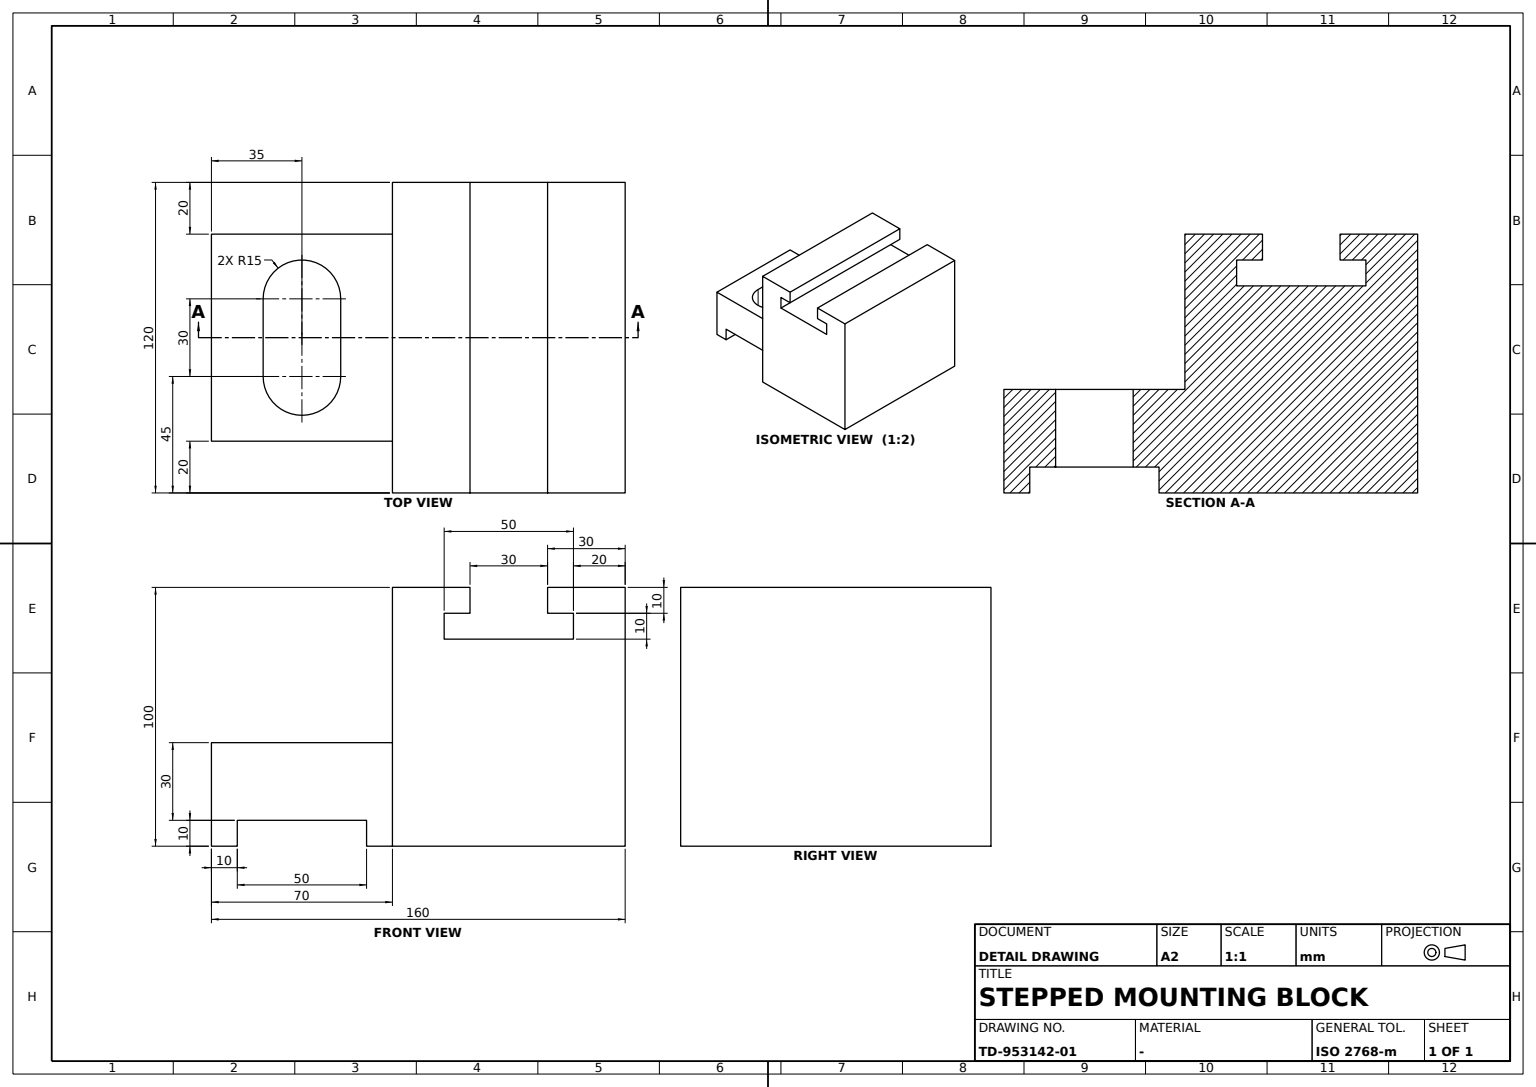
ISO-10303-21;
HEADER;
FILE_DESCRIPTION((''),'2;1');
FILE_NAME('','',(''),(''),'','','');
FILE_SCHEMA(('AUTOMOTIVE_DESIGN'));
ENDSEC;
DATA;
#1=APPLICATION_CONTEXT('');
#2=PRODUCT_CONTEXT('',#1,'mechanical');
#3=PRODUCT('','','',(#2));
#4=PRODUCT_DEFINITION_FORMATION('','',#3);
#5=PRODUCT_DEFINITION_CONTEXT('',#1,'design');
#6=PRODUCT_DEFINITION('','',#4,#5);
#7=PRODUCT_DEFINITION_SHAPE('','',#6);
#8=(LENGTH_UNIT()NAMED_UNIT(*)SI_UNIT(.MILLI.,.METRE.));
#9=(NAMED_UNIT(*)PLANE_ANGLE_UNIT()SI_UNIT($,.RADIAN.));
#10=(NAMED_UNIT(*)SI_UNIT($,.STERADIAN.)SOLID_ANGLE_UNIT());
#11=UNCERTAINTY_MEASURE_WITH_UNIT(LENGTH_MEASURE(1.E-05),#8,'distance_accuracy_value','');
#12=(GEOMETRIC_REPRESENTATION_CONTEXT(3)GLOBAL_UNCERTAINTY_ASSIGNED_CONTEXT((#11))GLOBAL_UNIT_ASSIGNED_CONTEXT((#8,#9,#10))REPRESENTATION_CONTEXT('',''));
#13=CARTESIAN_POINT('',(60.,70.,30.));
#14=VERTEX_POINT('',#13);
#15=CARTESIAN_POINT('',(60.,70.,40.));
#16=VERTEX_POINT('',#15);
#17=CARTESIAN_POINT('',(60.,70.,35.));
#18=DIRECTION('',(0.,0.,1.));
#19=VECTOR('',#18,1000.);
#20=LINE('',#17,#19);
#21=EDGE_CURVE('',#14,#16,#20,.T.);
#22=ORIENTED_EDGE('',*,*,#21,.T.);
#23=CARTESIAN_POINT('',(-60.,70.,40.));
#24=VERTEX_POINT('',#23);
#25=CARTESIAN_POINT('',(0.,70.,40.));
#26=DIRECTION('',(-1.,0.,0.));
#27=VECTOR('',#26,1000.);
#28=LINE('',#25,#27);
#29=EDGE_CURVE('',#16,#24,#28,.T.);
#30=ORIENTED_EDGE('',*,*,#29,.T.);
#31=CARTESIAN_POINT('',(-60.,70.,30.));
#32=VERTEX_POINT('',#31);
#33=CARTESIAN_POINT('',(-60.,70.,35.));
#34=LINE('',#33,#19);
#35=EDGE_CURVE('',#32,#24,#34,.T.);
#36=ORIENTED_EDGE('',*,*,#35,.F.);
#37=CARTESIAN_POINT('',(0.,70.,30.));
#38=LINE('',#37,#27);
#39=EDGE_CURVE('',#14,#32,#38,.T.);
#40=ORIENTED_EDGE('',*,*,#39,.F.);
#41=EDGE_LOOP('',(#22,#30,#36,#40));
#42=FACE_OUTER_BOUND('',#41,.T.);
#43=DIRECTION('',(0.,-1.,0.));
#44=AXIS2_PLACEMENT_3D('',#13,#43,#18);
#45=PLANE('',#44);
#46=ADVANCED_FACE('',(#42),#45,.T.);
#47=CARTESIAN_POINT('',(-15.,-20.,-40.));
#48=VERTEX_POINT('',#47);
#49=CARTESIAN_POINT('',(-15.,-50.,-40.));
#50=VERTEX_POINT('',#49);
#51=CARTESIAN_POINT('',(-15.,-35.,-40.));
#52=DIRECTION('',(0.,1.,0.));
#53=AXIS2_PLACEMENT_3D('',#51,#18,#52);
#54=CIRCLE('',#53,15.);
#55=EDGE_CURVE('',#48,#50,#54,.T.);
#56=ORIENTED_EDGE('',*,*,#55,.F.);
#57=CARTESIAN_POINT('',(-15.,-20.,-10.));
#58=VERTEX_POINT('',#57);
#59=CARTESIAN_POINT('',(-15.,-20.,-30.66));
#60=DIRECTION('',(0.,0.,-1.));
#61=VECTOR('',#60,1000.);
#62=LINE('',#59,#61);
#63=EDGE_CURVE('',#58,#48,#62,.T.);
#64=ORIENTED_EDGE('',*,*,#63,.F.);
#65=CARTESIAN_POINT('',(-15.,-50.,-10.));
#66=VERTEX_POINT('',#65);
#67=CARTESIAN_POINT('',(-15.,-35.,-10.));
#68=DIRECTION('',(1.,0.,0.));
#69=AXIS2_PLACEMENT_3D('',#67,#18,#68);
#70=CIRCLE('',#69,15.);
#71=EDGE_CURVE('',#58,#66,#70,.T.);
#72=ORIENTED_EDGE('',*,*,#71,.T.);
#73=CARTESIAN_POINT('',(-15.,-50.,-30.66));
#74=LINE('',#73,#61);
#75=EDGE_CURVE('',#66,#50,#74,.T.);
#76=ORIENTED_EDGE('',*,*,#75,.T.);
#77=EDGE_LOOP('',(#56,#64,#72,#76));
#78=FACE_OUTER_BOUND('',#77,.T.);
#79=CARTESIAN_POINT('',(-15.,-35.,-30.66));
#80=AXIS2_PLACEMENT_3D('',#79,#60,#68);
#81=CYLINDRICAL_SURFACE('',#80,15.);
#82=ADVANCED_FACE('',(#78),#81,.F.);
#83=CARTESIAN_POINT('',(40.,-70.,-50.));
#84=VERTEX_POINT('',#83);
#85=CARTESIAN_POINT('',(40.,-60.,-50.));
#86=VERTEX_POINT('',#85);
#87=CARTESIAN_POINT('',(40.,-65.,-50.));
#88=VECTOR('',#52,1000.);
#89=LINE('',#87,#88);
#90=EDGE_CURVE('',#84,#86,#89,.T.);
#91=ORIENTED_EDGE('',*,*,#90,.F.);
#92=CARTESIAN_POINT('',(-40.,-70.,-50.));
#93=VERTEX_POINT('',#92);
#94=CARTESIAN_POINT('',(0.,-70.,-50.));
#95=VECTOR('',#68,1000.);
#96=LINE('',#94,#95);
#97=EDGE_CURVE('',#93,#84,#96,.T.);
#98=ORIENTED_EDGE('',*,*,#97,.F.);
#99=CARTESIAN_POINT('',(-40.,-60.,-50.));
#100=VERTEX_POINT('',#99);
#101=CARTESIAN_POINT('',(-40.,-65.,-50.));
#102=LINE('',#101,#88);
#103=EDGE_CURVE('',#93,#100,#102,.T.);
#104=ORIENTED_EDGE('',*,*,#103,.T.);
#105=CARTESIAN_POINT('',(0.,-60.,-50.));
#106=LINE('',#105,#27);
#107=EDGE_CURVE('',#86,#100,#106,.T.);
#108=ORIENTED_EDGE('',*,*,#107,.F.);
#109=EDGE_LOOP('',(#91,#98,#104,#108));
#110=FACE_OUTER_BOUND('',#109,.T.);
#111=CARTESIAN_POINT('',(0.,90.,-50.));
#112=AXIS2_PLACEMENT_3D('',#111,#18,#43);
#113=PLANE('',#112);
#114=ADVANCED_FACE('',(#110),#113,.F.);
#115=CARTESIAN_POINT('',(30.,-35.,-10.));
#116=VERTEX_POINT('',#115);
#117=CARTESIAN_POINT('',(30.,-35.,-40.));
#118=VERTEX_POINT('',#117);
#119=CARTESIAN_POINT('',(30.,-35.,-30.66));
#120=LINE('',#119,#61);
#121=EDGE_CURVE('',#116,#118,#120,.T.);
#122=ORIENTED_EDGE('',*,*,#121,.T.);
#123=CARTESIAN_POINT('',(15.,-50.,-40.));
#124=VERTEX_POINT('',#123);
#125=CARTESIAN_POINT('',(15.,-35.,-40.));
#126=AXIS2_PLACEMENT_3D('',#125,#18,#52);
#127=CIRCLE('',#126,15.);
#128=EDGE_CURVE('',#124,#118,#127,.T.);
#129=ORIENTED_EDGE('',*,*,#128,.F.);
#130=CARTESIAN_POINT('',(15.,-50.,-10.));
#131=VERTEX_POINT('',#130);
#132=CARTESIAN_POINT('',(15.,-50.,-25.));
#133=LINE('',#132,#61);
#134=EDGE_CURVE('',#131,#124,#133,.T.);
#135=ORIENTED_EDGE('',*,*,#134,.F.);
#136=CARTESIAN_POINT('',(15.,-35.,-10.));
#137=AXIS2_PLACEMENT_3D('',#136,#18,#68);
#138=CIRCLE('',#137,15.);
#139=EDGE_CURVE('',#131,#116,#138,.T.);
#140=ORIENTED_EDGE('',*,*,#139,.T.);
#141=EDGE_LOOP('',(#122,#129,#135,#140));
#142=FACE_OUTER_BOUND('',#141,.T.);
#143=CARTESIAN_POINT('',(15.,-35.,-30.66));
#144=AXIS2_PLACEMENT_3D('',#143,#60,#68);
#145=CYLINDRICAL_SURFACE('',#144,15.);
#146=ADVANCED_FACE('',(#142),#145,.F.);
#147=ORIENTED_EDGE('',*,*,#55,.T.);
#148=CARTESIAN_POINT('',(0.,-50.,-40.));
#149=LINE('',#148,#27);
#150=EDGE_CURVE('',#124,#50,#149,.T.);
#151=ORIENTED_EDGE('',*,*,#150,.F.);
#152=ORIENTED_EDGE('',*,*,#128,.T.);
#153=CARTESIAN_POINT('',(15.,-20.,-40.));
#154=VERTEX_POINT('',#153);
#155=EDGE_CURVE('',#118,#154,#127,.T.);
#156=ORIENTED_EDGE('',*,*,#155,.T.);
#157=CARTESIAN_POINT('',(0.,-20.,-40.));
#158=LINE('',#157,#95);
#159=EDGE_CURVE('',#48,#154,#158,.T.);
#160=ORIENTED_EDGE('',*,*,#159,.F.);
#161=EDGE_LOOP('',(#147,#151,#152,#156,#160));
#162=FACE_BOUND('',#161,.T.);
#163=CARTESIAN_POINT('',(40.,-10.,-40.));
#164=VERTEX_POINT('',#163);
#165=CARTESIAN_POINT('',(-40.,-10.,-40.));
#166=VERTEX_POINT('',#165);
#167=CARTESIAN_POINT('',(0.,-10.,-40.));
#168=LINE('',#167,#27);
#169=EDGE_CURVE('',#164,#166,#168,.T.);
#170=ORIENTED_EDGE('',*,*,#169,.F.);
#171=CARTESIAN_POINT('',(40.,-60.,-40.));
#172=VERTEX_POINT('',#171);
#173=CARTESIAN_POINT('',(40.,-35.,-40.));
#174=VECTOR('',#43,1000.);
#175=LINE('',#173,#174);
#176=EDGE_CURVE('',#164,#172,#175,.T.);
#177=ORIENTED_EDGE('',*,*,#176,.T.);
#178=CARTESIAN_POINT('',(-40.,-60.,-40.));
#179=VERTEX_POINT('',#178);
#180=CARTESIAN_POINT('',(0.,-60.,-40.));
#181=LINE('',#180,#27);
#182=EDGE_CURVE('',#172,#179,#181,.T.);
#183=ORIENTED_EDGE('',*,*,#182,.T.);
#184=CARTESIAN_POINT('',(-40.,-35.,-40.));
#185=LINE('',#184,#88);
#186=EDGE_CURVE('',#179,#166,#185,.T.);
#187=ORIENTED_EDGE('',*,*,#186,.T.);
#188=EDGE_LOOP('',(#170,#177,#183,#187));
#189=FACE_OUTER_BOUND('',#188,.T.);
#190=AXIS2_PLACEMENT_3D('',#171,#18,#52);
#191=PLANE('',#190);
#192=ADVANCED_FACE('',(#162,#189),#191,.F.);
#193=CARTESIAN_POINT('',(15.,-20.,-10.));
#194=VERTEX_POINT('',#193);
#195=CARTESIAN_POINT('',(0.,-20.,-10.));
#196=LINE('',#195,#27);
#197=EDGE_CURVE('',#194,#58,#196,.T.);
#198=ORIENTED_EDGE('',*,*,#197,.F.);
#199=EDGE_CURVE('',#116,#194,#138,.T.);
#200=ORIENTED_EDGE('',*,*,#199,.F.);
#201=ORIENTED_EDGE('',*,*,#139,.F.);
#202=CARTESIAN_POINT('',(0.,-50.,-10.));
#203=LINE('',#202,#95);
#204=EDGE_CURVE('',#66,#131,#203,.T.);
#205=ORIENTED_EDGE('',*,*,#204,.F.);
#206=ORIENTED_EDGE('',*,*,#71,.F.);
#207=EDGE_LOOP('',(#198,#200,#201,#205,#206));
#208=FACE_BOUND('',#207,.T.);
#209=CARTESIAN_POINT('',(-40.,0.,-10.));
#210=VERTEX_POINT('',#209);
#211=CARTESIAN_POINT('',(-40.,-70.,-10.));
#212=VERTEX_POINT('',#211);
#213=CARTESIAN_POINT('',(-40.,-35.,-10.));
#214=LINE('',#213,#174);
#215=EDGE_CURVE('',#210,#212,#214,.T.);
#216=ORIENTED_EDGE('',*,*,#215,.T.);
#217=CARTESIAN_POINT('',(40.,-70.,-10.));
#218=VERTEX_POINT('',#217);
#219=CARTESIAN_POINT('',(0.,-70.,-10.));
#220=LINE('',#219,#95);
#221=EDGE_CURVE('',#212,#218,#220,.T.);
#222=ORIENTED_EDGE('',*,*,#221,.T.);
#223=CARTESIAN_POINT('',(40.,0.,-10.));
#224=VERTEX_POINT('',#223);
#225=CARTESIAN_POINT('',(40.,-35.,-10.));
#226=LINE('',#225,#174);
#227=EDGE_CURVE('',#224,#218,#226,.T.);
#228=ORIENTED_EDGE('',*,*,#227,.F.);
#229=CARTESIAN_POINT('',(0.,0.,-10.));
#230=LINE('',#229,#95);
#231=EDGE_CURVE('',#210,#224,#230,.T.);
#232=ORIENTED_EDGE('',*,*,#231,.F.);
#233=EDGE_LOOP('',(#216,#222,#228,#232));
#234=FACE_OUTER_BOUND('',#233,.T.);
#235=AXIS2_PLACEMENT_3D('',#229,#18,#43);
#236=PLANE('',#235);
#237=ADVANCED_FACE('',(#208,#234),#236,.T.);
#238=CARTESIAN_POINT('',(-60.,0.,50.));
#239=VERTEX_POINT('',#238);
#240=CARTESIAN_POINT('',(60.,0.,50.));
#241=VERTEX_POINT('',#240);
#242=CARTESIAN_POINT('',(0.,0.,50.));
#243=LINE('',#242,#95);
#244=EDGE_CURVE('',#239,#241,#243,.T.);
#245=ORIENTED_EDGE('',*,*,#244,.T.);
#246=CARTESIAN_POINT('',(60.,30.,50.));
#247=VERTEX_POINT('',#246);
#248=CARTESIAN_POINT('',(60.,15.,50.));
#249=LINE('',#248,#174);
#250=EDGE_CURVE('',#247,#241,#249,.T.);
#251=ORIENTED_EDGE('',*,*,#250,.F.);
#252=CARTESIAN_POINT('',(-60.,30.,50.));
#253=VERTEX_POINT('',#252);
#254=CARTESIAN_POINT('',(0.,30.,50.));
#255=LINE('',#254,#27);
#256=EDGE_CURVE('',#247,#253,#255,.T.);
#257=ORIENTED_EDGE('',*,*,#256,.T.);
#258=CARTESIAN_POINT('',(-60.,15.,50.));
#259=LINE('',#258,#174);
#260=EDGE_CURVE('',#253,#239,#259,.T.);
#261=ORIENTED_EDGE('',*,*,#260,.T.);
#262=EDGE_LOOP('',(#245,#251,#257,#261));
#263=FACE_OUTER_BOUND('',#262,.T.);
#264=AXIS2_PLACEMENT_3D('',#242,#60,#52);
#265=PLANE('',#264);
#266=ADVANCED_FACE('',(#263),#265,.F.);
#267=CARTESIAN_POINT('',(60.,60.,50.));
#268=VERTEX_POINT('',#267);
#269=CARTESIAN_POINT('',(-60.,60.,50.));
#270=VERTEX_POINT('',#269);
#271=CARTESIAN_POINT('',(0.,60.,50.));
#272=LINE('',#271,#27);
#273=EDGE_CURVE('',#268,#270,#272,.T.);
#274=ORIENTED_EDGE('',*,*,#273,.F.);
#275=CARTESIAN_POINT('',(60.,90.,50.));
#276=VERTEX_POINT('',#275);
#277=CARTESIAN_POINT('',(60.,75.,50.));
#278=LINE('',#277,#174);
#279=EDGE_CURVE('',#276,#268,#278,.T.);
#280=ORIENTED_EDGE('',*,*,#279,.F.);
#281=CARTESIAN_POINT('',(-60.,90.,50.));
#282=VERTEX_POINT('',#281);
#283=CARTESIAN_POINT('',(0.,90.,50.));
#284=LINE('',#283,#95);
#285=EDGE_CURVE('',#282,#276,#284,.T.);
#286=ORIENTED_EDGE('',*,*,#285,.F.);
#287=CARTESIAN_POINT('',(-60.,75.,50.));
#288=LINE('',#287,#174);
#289=EDGE_CURVE('',#282,#270,#288,.T.);
#290=ORIENTED_EDGE('',*,*,#289,.T.);
#291=EDGE_LOOP('',(#274,#280,#286,#290));
#292=FACE_OUTER_BOUND('',#291,.T.);
#293=ADVANCED_FACE('',(#292),#265,.F.);
#294=ORIENTED_EDGE('',*,*,#285,.T.);
#295=CARTESIAN_POINT('',(60.,90.,-50.));
#296=VERTEX_POINT('',#295);
#297=CARTESIAN_POINT('',(60.,90.,0.));
#298=LINE('',#297,#19);
#299=EDGE_CURVE('',#296,#276,#298,.T.);
#300=ORIENTED_EDGE('',*,*,#299,.F.);
#301=CARTESIAN_POINT('',(-60.,90.,-50.));
#302=VERTEX_POINT('',#301);
#303=LINE('',#111,#95);
#304=EDGE_CURVE('',#302,#296,#303,.T.);
#305=ORIENTED_EDGE('',*,*,#304,.F.);
#306=CARTESIAN_POINT('',(-60.,90.,0.));
#307=LINE('',#306,#19);
#308=EDGE_CURVE('',#302,#282,#307,.T.);
#309=ORIENTED_EDGE('',*,*,#308,.T.);
#310=EDGE_LOOP('',(#294,#300,#305,#309));
#311=FACE_OUTER_BOUND('',#310,.T.);
#312=AXIS2_PLACEMENT_3D('',#283,#43,#60);
#313=PLANE('',#312);
#314=ADVANCED_FACE('',(#311),#313,.F.);
#315=ORIENTED_EDGE('',*,*,#159,.T.);
#316=CARTESIAN_POINT('',(15.,-20.,-30.66));
#317=LINE('',#316,#61);
#318=EDGE_CURVE('',#194,#154,#317,.T.);
#319=ORIENTED_EDGE('',*,*,#318,.F.);
#320=ORIENTED_EDGE('',*,*,#197,.T.);
#321=ORIENTED_EDGE('',*,*,#63,.T.);
#322=EDGE_LOOP('',(#315,#319,#320,#321));
#323=FACE_OUTER_BOUND('',#322,.T.);
#324=AXIS2_PLACEMENT_3D('',#57,#52,#68);
#325=PLANE('',#324);
#326=ADVANCED_FACE('',(#323),#325,.F.);
#327=CARTESIAN_POINT('',(-60.,20.,30.));
#328=VERTEX_POINT('',#327);
#329=CARTESIAN_POINT('',(-60.,45.,30.));
#330=LINE('',#329,#88);
#331=EDGE_CURVE('',#328,#32,#330,.T.);
#332=ORIENTED_EDGE('',*,*,#331,.F.);
#333=CARTESIAN_POINT('',(60.,20.,30.));
#334=VERTEX_POINT('',#333);
#335=CARTESIAN_POINT('',(0.,20.,30.));
#336=LINE('',#335,#27);
#337=EDGE_CURVE('',#334,#328,#336,.T.);
#338=ORIENTED_EDGE('',*,*,#337,.F.);
#339=CARTESIAN_POINT('',(60.,45.,30.));
#340=LINE('',#339,#88);
#341=EDGE_CURVE('',#334,#14,#340,.T.);
#342=ORIENTED_EDGE('',*,*,#341,.T.);
#343=ORIENTED_EDGE('',*,*,#39,.T.);
#344=EDGE_LOOP('',(#332,#338,#342,#343));
#345=FACE_OUTER_BOUND('',#344,.T.);
#346=AXIS2_PLACEMENT_3D('',#333,#18,#52);
#347=PLANE('',#346);
#348=ADVANCED_FACE('',(#345),#347,.T.);
#349=CARTESIAN_POINT('',(-60.,30.,40.));
#350=VERTEX_POINT('',#349);
#351=CARTESIAN_POINT('',(-60.,30.,45.));
#352=LINE('',#351,#61);
#353=EDGE_CURVE('',#253,#350,#352,.T.);
#354=ORIENTED_EDGE('',*,*,#353,.T.);
#355=CARTESIAN_POINT('',(-60.,20.,40.));
#356=VERTEX_POINT('',#355);
#357=CARTESIAN_POINT('',(-60.,25.,40.));
#358=LINE('',#357,#174);
#359=EDGE_CURVE('',#350,#356,#358,.T.);
#360=ORIENTED_EDGE('',*,*,#359,.T.);
#361=CARTESIAN_POINT('',(-60.,20.,35.));
#362=LINE('',#361,#61);
#363=EDGE_CURVE('',#356,#328,#362,.T.);
#364=ORIENTED_EDGE('',*,*,#363,.T.);
#365=ORIENTED_EDGE('',*,*,#331,.T.);
#366=ORIENTED_EDGE('',*,*,#35,.T.);
#367=CARTESIAN_POINT('',(-60.,60.,40.));
#368=VERTEX_POINT('',#367);
#369=CARTESIAN_POINT('',(-60.,65.,40.));
#370=LINE('',#369,#174);
#371=EDGE_CURVE('',#24,#368,#370,.T.);
#372=ORIENTED_EDGE('',*,*,#371,.T.);
#373=CARTESIAN_POINT('',(-60.,60.,45.));
#374=LINE('',#373,#61);
#375=EDGE_CURVE('',#270,#368,#374,.T.);
#376=ORIENTED_EDGE('',*,*,#375,.F.);
#377=ORIENTED_EDGE('',*,*,#289,.F.);
#378=ORIENTED_EDGE('',*,*,#308,.F.);
#379=CARTESIAN_POINT('',(-60.,0.,-50.));
#380=VERTEX_POINT('',#379);
#381=CARTESIAN_POINT('',(-60.,45.,-50.));
#382=LINE('',#381,#88);
#383=EDGE_CURVE('',#380,#302,#382,.T.);
#384=ORIENTED_EDGE('',*,*,#383,.F.);
#385=CARTESIAN_POINT('',(-60.,0.,0.));
#386=LINE('',#385,#61);
#387=EDGE_CURVE('',#239,#380,#386,.T.);
#388=ORIENTED_EDGE('',*,*,#387,.F.);
#389=ORIENTED_EDGE('',*,*,#260,.F.);
#390=EDGE_LOOP('',(#354,#360,#364,#365,#366,#372,#376,#377,#378,#384,#388,#389));
#391=FACE_OUTER_BOUND('',#390,.T.);
#392=AXIS2_PLACEMENT_3D('',#385,#68,#52);
#393=PLANE('',#392);
#394=ADVANCED_FACE('',(#391),#393,.F.);
#395=ORIENTED_EDGE('',*,*,#182,.F.);
#396=CARTESIAN_POINT('',(40.,-60.,-45.));
#397=LINE('',#396,#61);
#398=EDGE_CURVE('',#172,#86,#397,.T.);
#399=ORIENTED_EDGE('',*,*,#398,.T.);
#400=ORIENTED_EDGE('',*,*,#107,.T.);
#401=CARTESIAN_POINT('',(-40.,-60.,-45.));
#402=LINE('',#401,#61);
#403=EDGE_CURVE('',#179,#100,#402,.T.);
#404=ORIENTED_EDGE('',*,*,#403,.F.);
#405=EDGE_LOOP('',(#395,#399,#400,#404));
#406=FACE_OUTER_BOUND('',#405,.T.);
#407=AXIS2_PLACEMENT_3D('',#171,#52,#60);
#408=PLANE('',#407);
#409=ADVANCED_FACE('',(#406),#408,.T.);
#410=CARTESIAN_POINT('',(-40.,0.,-50.));
#411=VERTEX_POINT('',#410);
#412=CARTESIAN_POINT('',(-40.,0.,-30.));
#413=LINE('',#412,#19);
#414=EDGE_CURVE('',#411,#210,#413,.T.);
#415=ORIENTED_EDGE('',*,*,#414,.F.);
#416=CARTESIAN_POINT('',(-40.,-10.,-50.));
#417=VERTEX_POINT('',#416);
#418=CARTESIAN_POINT('',(-40.,-5.,-50.));
#419=LINE('',#418,#88);
#420=EDGE_CURVE('',#417,#411,#419,.T.);
#421=ORIENTED_EDGE('',*,*,#420,.F.);
#422=CARTESIAN_POINT('',(-40.,-10.,-45.));
#423=LINE('',#422,#61);
#424=EDGE_CURVE('',#166,#417,#423,.T.);
#425=ORIENTED_EDGE('',*,*,#424,.F.);
#426=ORIENTED_EDGE('',*,*,#186,.F.);
#427=ORIENTED_EDGE('',*,*,#403,.T.);
#428=ORIENTED_EDGE('',*,*,#103,.F.);
#429=CARTESIAN_POINT('',(-40.,-70.,-30.));
#430=LINE('',#429,#61);
#431=EDGE_CURVE('',#212,#93,#430,.T.);
#432=ORIENTED_EDGE('',*,*,#431,.F.);
#433=ORIENTED_EDGE('',*,*,#215,.F.);
#434=EDGE_LOOP('',(#415,#421,#425,#426,#427,#428,#432,#433));
#435=FACE_OUTER_BOUND('',#434,.T.);
#436=CARTESIAN_POINT('',(-40.,0.,0.));
#437=AXIS2_PLACEMENT_3D('',#436,#68,#52);
#438=PLANE('',#437);
#439=ADVANCED_FACE('',(#435),#438,.F.);
#440=CARTESIAN_POINT('',(60.,0.,-50.));
#441=VERTEX_POINT('',#440);
#442=CARTESIAN_POINT('',(60.,0.,0.));
#443=LINE('',#442,#61);
#444=EDGE_CURVE('',#241,#441,#443,.T.);
#445=ORIENTED_EDGE('',*,*,#444,.F.);
#446=ORIENTED_EDGE('',*,*,#244,.F.);
#447=ORIENTED_EDGE('',*,*,#387,.T.);
#448=CARTESIAN_POINT('',(-50.,0.,-50.));
#449=LINE('',#448,#95);
#450=EDGE_CURVE('',#380,#411,#449,.T.);
#451=ORIENTED_EDGE('',*,*,#450,.T.);
#452=ORIENTED_EDGE('',*,*,#414,.T.);
#453=ORIENTED_EDGE('',*,*,#231,.T.);
#454=CARTESIAN_POINT('',(40.,0.,-50.));
#455=VERTEX_POINT('',#454);
#456=CARTESIAN_POINT('',(40.,0.,-30.));
#457=LINE('',#456,#19);
#458=EDGE_CURVE('',#455,#224,#457,.T.);
#459=ORIENTED_EDGE('',*,*,#458,.F.);
#460=CARTESIAN_POINT('',(50.,0.,-50.));
#461=LINE('',#460,#95);
#462=EDGE_CURVE('',#455,#441,#461,.T.);
#463=ORIENTED_EDGE('',*,*,#462,.T.);
#464=EDGE_LOOP('',(#445,#446,#447,#451,#452,#453,#459,#463));
#465=FACE_OUTER_BOUND('',#464,.T.);
#466=AXIS2_PLACEMENT_3D('',#242,#43,#60);
#467=PLANE('',#466);
#468=ADVANCED_FACE('',(#465),#467,.T.);
#469=ORIENTED_EDGE('',*,*,#458,.T.);
#470=ORIENTED_EDGE('',*,*,#227,.T.);
#471=CARTESIAN_POINT('',(40.,-70.,-30.));
#472=LINE('',#471,#61);
#473=EDGE_CURVE('',#218,#84,#472,.T.);
#474=ORIENTED_EDGE('',*,*,#473,.T.);
#475=ORIENTED_EDGE('',*,*,#90,.T.);
#476=ORIENTED_EDGE('',*,*,#398,.F.);
#477=ORIENTED_EDGE('',*,*,#176,.F.);
#478=CARTESIAN_POINT('',(40.,-10.,-50.));
#479=VERTEX_POINT('',#478);
#480=CARTESIAN_POINT('',(40.,-10.,-45.));
#481=LINE('',#480,#19);
#482=EDGE_CURVE('',#479,#164,#481,.T.);
#483=ORIENTED_EDGE('',*,*,#482,.F.);
#484=CARTESIAN_POINT('',(40.,-5.,-50.));
#485=LINE('',#484,#88);
#486=EDGE_CURVE('',#479,#455,#485,.T.);
#487=ORIENTED_EDGE('',*,*,#486,.T.);
#488=EDGE_LOOP('',(#469,#470,#474,#475,#476,#477,#483,#487));
#489=FACE_OUTER_BOUND('',#488,.T.);
#490=CARTESIAN_POINT('',(40.,0.,0.));
#491=AXIS2_PLACEMENT_3D('',#490,#68,#52);
#492=PLANE('',#491);
#493=ADVANCED_FACE('',(#489),#492,.T.);
#494=ORIENTED_EDGE('',*,*,#304,.T.);
#495=CARTESIAN_POINT('',(60.,45.,-50.));
#496=LINE('',#495,#88);
#497=EDGE_CURVE('',#441,#296,#496,.T.);
#498=ORIENTED_EDGE('',*,*,#497,.F.);
#499=ORIENTED_EDGE('',*,*,#462,.F.);
#500=ORIENTED_EDGE('',*,*,#486,.F.);
#501=CARTESIAN_POINT('',(0.,-10.,-50.));
#502=LINE('',#501,#27);
#503=EDGE_CURVE('',#479,#417,#502,.T.);
#504=ORIENTED_EDGE('',*,*,#503,.T.);
#505=ORIENTED_EDGE('',*,*,#420,.T.);
#506=ORIENTED_EDGE('',*,*,#450,.F.);
#507=ORIENTED_EDGE('',*,*,#383,.T.);
#508=EDGE_LOOP('',(#494,#498,#499,#500,#504,#505,#506,#507));
#509=FACE_OUTER_BOUND('',#508,.T.);
#510=ADVANCED_FACE('',(#509),#113,.F.);
#511=ORIENTED_EDGE('',*,*,#97,.T.);
#512=ORIENTED_EDGE('',*,*,#473,.F.);
#513=ORIENTED_EDGE('',*,*,#221,.F.);
#514=ORIENTED_EDGE('',*,*,#431,.T.);
#515=EDGE_LOOP('',(#511,#512,#513,#514));
#516=FACE_OUTER_BOUND('',#515,.T.);
#517=AXIS2_PLACEMENT_3D('',#219,#43,#60);
#518=PLANE('',#517);
#519=ADVANCED_FACE('',(#516),#518,.T.);
#520=ORIENTED_EDGE('',*,*,#318,.T.);
#521=ORIENTED_EDGE('',*,*,#155,.F.);
#522=ORIENTED_EDGE('',*,*,#121,.F.);
#523=ORIENTED_EDGE('',*,*,#199,.T.);
#524=EDGE_LOOP('',(#520,#521,#522,#523));
#525=FACE_OUTER_BOUND('',#524,.T.);
#526=ADVANCED_FACE('',(#525),#145,.F.);
#527=ORIENTED_EDGE('',*,*,#341,.F.);
#528=CARTESIAN_POINT('',(60.,20.,40.));
#529=VERTEX_POINT('',#528);
#530=CARTESIAN_POINT('',(60.,20.,35.));
#531=LINE('',#530,#61);
#532=EDGE_CURVE('',#529,#334,#531,.T.);
#533=ORIENTED_EDGE('',*,*,#532,.F.);
#534=CARTESIAN_POINT('',(60.,30.,40.));
#535=VERTEX_POINT('',#534);
#536=CARTESIAN_POINT('',(60.,25.,40.));
#537=LINE('',#536,#174);
#538=EDGE_CURVE('',#535,#529,#537,.T.);
#539=ORIENTED_EDGE('',*,*,#538,.F.);
#540=CARTESIAN_POINT('',(60.,30.,45.));
#541=LINE('',#540,#61);
#542=EDGE_CURVE('',#247,#535,#541,.T.);
#543=ORIENTED_EDGE('',*,*,#542,.F.);
#544=ORIENTED_EDGE('',*,*,#250,.T.);
#545=ORIENTED_EDGE('',*,*,#444,.T.);
#546=ORIENTED_EDGE('',*,*,#497,.T.);
#547=ORIENTED_EDGE('',*,*,#299,.T.);
#548=ORIENTED_EDGE('',*,*,#279,.T.);
#549=CARTESIAN_POINT('',(60.,60.,40.));
#550=VERTEX_POINT('',#549);
#551=CARTESIAN_POINT('',(60.,60.,45.));
#552=LINE('',#551,#19);
#553=EDGE_CURVE('',#550,#268,#552,.T.);
#554=ORIENTED_EDGE('',*,*,#553,.F.);
#555=CARTESIAN_POINT('',(60.,65.,40.));
#556=LINE('',#555,#174);
#557=EDGE_CURVE('',#16,#550,#556,.T.);
#558=ORIENTED_EDGE('',*,*,#557,.F.);
#559=ORIENTED_EDGE('',*,*,#21,.F.);
#560=EDGE_LOOP('',(#527,#533,#539,#543,#544,#545,#546,#547,#548,#554,#558,#559));
#561=FACE_OUTER_BOUND('',#560,.T.);
#562=AXIS2_PLACEMENT_3D('',#442,#68,#52);
#563=PLANE('',#562);
#564=ADVANCED_FACE('',(#561),#563,.T.);
#565=ORIENTED_EDGE('',*,*,#532,.T.);
#566=ORIENTED_EDGE('',*,*,#337,.T.);
#567=ORIENTED_EDGE('',*,*,#363,.F.);
#568=CARTESIAN_POINT('',(0.,20.,40.));
#569=LINE('',#568,#27);
#570=EDGE_CURVE('',#529,#356,#569,.T.);
#571=ORIENTED_EDGE('',*,*,#570,.F.);
#572=EDGE_LOOP('',(#565,#566,#567,#571));
#573=FACE_OUTER_BOUND('',#572,.T.);
#574=AXIS2_PLACEMENT_3D('',#528,#52,#60);
#575=PLANE('',#574);
#576=ADVANCED_FACE('',(#573),#575,.T.);
#577=CARTESIAN_POINT('',(0.,30.,40.));
#578=LINE('',#577,#27);
#579=EDGE_CURVE('',#535,#350,#578,.T.);
#580=ORIENTED_EDGE('',*,*,#579,.F.);
#581=ORIENTED_EDGE('',*,*,#538,.T.);
#582=ORIENTED_EDGE('',*,*,#570,.T.);
#583=ORIENTED_EDGE('',*,*,#359,.F.);
#584=EDGE_LOOP('',(#580,#581,#582,#583));
#585=FACE_OUTER_BOUND('',#584,.T.);
#586=AXIS2_PLACEMENT_3D('',#534,#60,#43);
#587=PLANE('',#586);
#588=ADVANCED_FACE('',(#585),#587,.T.);
#589=ORIENTED_EDGE('',*,*,#150,.T.);
#590=ORIENTED_EDGE('',*,*,#75,.F.);
#591=ORIENTED_EDGE('',*,*,#204,.T.);
#592=ORIENTED_EDGE('',*,*,#134,.T.);
#593=EDGE_LOOP('',(#589,#590,#591,#592));
#594=FACE_OUTER_BOUND('',#593,.T.);
#595=AXIS2_PLACEMENT_3D('',#130,#43,#26);
#596=PLANE('',#595);
#597=ADVANCED_FACE('',(#594),#596,.F.);
#598=ORIENTED_EDGE('',*,*,#371,.F.);
#599=ORIENTED_EDGE('',*,*,#29,.F.);
#600=ORIENTED_EDGE('',*,*,#557,.T.);
#601=CARTESIAN_POINT('',(0.,60.,40.));
#602=LINE('',#601,#27);
#603=EDGE_CURVE('',#550,#368,#602,.T.);
#604=ORIENTED_EDGE('',*,*,#603,.T.);
#605=EDGE_LOOP('',(#598,#599,#600,#604));
#606=FACE_OUTER_BOUND('',#605,.T.);
#607=ADVANCED_FACE('',(#606),#587,.T.);
#608=ORIENTED_EDGE('',*,*,#169,.T.);
#609=ORIENTED_EDGE('',*,*,#424,.T.);
#610=ORIENTED_EDGE('',*,*,#503,.F.);
#611=ORIENTED_EDGE('',*,*,#482,.T.);
#612=EDGE_LOOP('',(#608,#609,#610,#611));
#613=FACE_OUTER_BOUND('',#612,.T.);
#614=CARTESIAN_POINT('',(40.,-10.,-55.178875));
#615=AXIS2_PLACEMENT_3D('',#614,#43,#18);
#616=PLANE('',#615);
#617=ADVANCED_FACE('',(#613),#616,.T.);
#618=ORIENTED_EDGE('',*,*,#553,.T.);
#619=ORIENTED_EDGE('',*,*,#273,.T.);
#620=ORIENTED_EDGE('',*,*,#375,.T.);
#621=ORIENTED_EDGE('',*,*,#603,.F.);
#622=EDGE_LOOP('',(#618,#619,#620,#621));
#623=FACE_OUTER_BOUND('',#622,.T.);
#624=AXIS2_PLACEMENT_3D('',#549,#43,#18);
#625=PLANE('',#624);
#626=ADVANCED_FACE('',(#623),#625,.T.);
#627=ORIENTED_EDGE('',*,*,#542,.T.);
#628=ORIENTED_EDGE('',*,*,#579,.T.);
#629=ORIENTED_EDGE('',*,*,#353,.F.);
#630=ORIENTED_EDGE('',*,*,#256,.F.);
#631=EDGE_LOOP('',(#627,#628,#629,#630));
#632=FACE_OUTER_BOUND('',#631,.T.);
#633=AXIS2_PLACEMENT_3D('',#246,#52,#60);
#634=PLANE('',#633);
#635=ADVANCED_FACE('',(#632),#634,.T.);
#636=CLOSED_SHELL('',(#46,#82,#114,#146,#192,#237,#266,#293,#314,#326,#348,#394,#409,#439,#468,#493,#510,#519,#526,#564,#576,#588,#597,#607,#617,#626,#635));
#637=MANIFOLD_SOLID_BREP('',#636);
#638=ADVANCED_BREP_SHAPE_REPRESENTATION('',(#637),#12);
#639=SHAPE_DEFINITION_REPRESENTATION(#7,#638);
ENDSEC;
END-ISO-10303-21;
